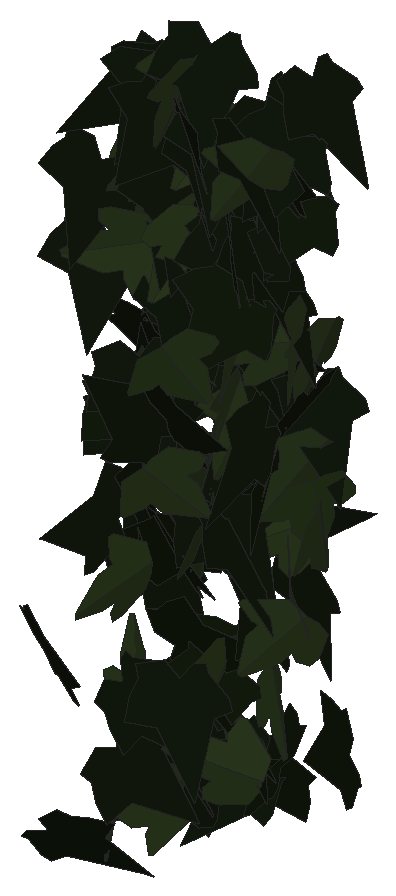
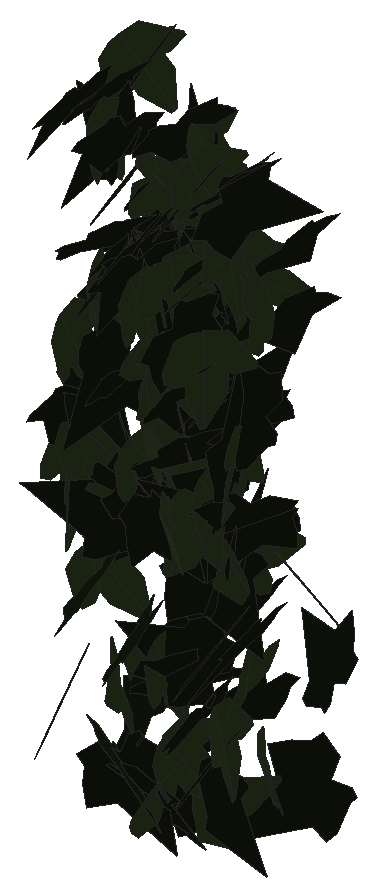
# SketchUp Ruby script. Lengths in inches.
U = 1.inch
M = Sketchup.active_model
def pt(a) = Geom::Point3d.new(a.map { |v| v * U })
def face(e, loops, mat)
  f = e.add_face(loops[0].map { |a| pt(a) })
  loops[1..].each { |l| e.add_face(l.map { |a| pt(a) }).erase! }
  f.material = f.back_material = mat if mat
  f
end
# faces: each face lists its corners as indices into pts; further lists are holes
def faces(e, pts, list, mat = nil) = list.each { |f| face(e, (f[0].is_a?(Array) ? f : [f]).map { |l| l.map { |i| pts[i] } }, mat) }
# xy, xz, yz: faces in a plane at the given z, y or x. An outline is a flat list of corners, or four numbers for a rectangle; further outlines are holes
def ring(l) = l.size == 4 ? [[l[0], l[1]], [l[2], l[1]], [l[2], l[3]], [l[0], l[3]]] : l.each_slice(2).to_a
def flat(e, list, mat, &to3) = list.each { |f| face(e, (f[0].is_a?(Array) ? f : [f]).map { |l| ring(l).map { |u, v| to3.(u, v) } }, mat) }
def xy(e, z, list, mat = nil) = flat(e, list, mat) { |x, y| [x, y, z] }
def xz(e, y, list, mat = nil) = flat(e, list, mat) { |x, z| [x, y, z] }
def yz(e, x, list, mat = nil) = flat(e, list, mat) { |y, z| [x, y, z] }
def lines(e, pts, list) = list.each { |a, b| e.add_line(pt(pts[a]), pt(pts[b])) }
# prism: a flat outline (further loops are holes) pulled along v
def prism(e, loops, v, mat = nil)
  f = face(e, loops, mat); d = Geom::Vector3d.new(v.map { |x| x * U })
  f.pushpull(f.normal.samedirection?(d) ? d.length : -d.length)
end
def box(e, o, s, mat = nil) = prism(e, [[o, [o[0] + s[0], o[1], o[2]], [o[0] + s[0], o[1] + s[1], o[2]], [o[0], o[1] + s[1], o[2]]]], [0, 0, s[2]], mat)
def at(x, y, z, deg = 0) = Geom::Transformation.translation(pt([x, y, z])) * Geom::Transformation.rotation(ORIGIN, Z_AXIS, deg.degrees)
def axes(o, x, y, z) = Geom::Transformation.new([*x, 0, *y, 0, *z, 0, *pt(o).to_a, 1])
def part(name) = M.definitions.add(name)
# library, detail: a bought-in or finely detailed component or shape, given as its bounding box
def library(name, o, s) = part(name).tap { |d| box(d.entities, o, s) }
def detail(e, o, s) = box(e.add_group.entities, o, s)
def put(e, d, t, mat = nil) = e.add_instance(d, t).tap { |i| i.material = mat if mat }
def group(e, t, mat = nil) = e.add_group.tap { |g| g.transformation = t; g.material = mat if mat }.entities
root = M.entities
M.materials.add("efeu1").color = [18, 25, 13]
M.materials.add("efeu2").color = [43, 57, 29]
c1 = part("ivyleaf_10")
p = [[0,0.5,-0.03],[-0.0625,2.02,-0.43],[-0.19,2.01,-0.46],[-0.54,1.05,-0.29],[-0.52,0.625,-0.18],[-0.83,0.76,-0.28],
  [-1.16,0.64,-0.33],[-1.15,0.33,-0.24],[-0.77,-0.39,0.02],[-0.3,-0.51,0.16],[0.04,-0.48,0.23],[-0.02,2.01,-0.4375],
  [-0.06,2.01,-0.43],[0.04,-0.49,0.23],[0.67,-0.49,0.14],[1.38,0.36,-0.2],[1.375,0.51,-0.24],[0.81,0.65,-0.19],
  [0.62,0.59,-0.15],[0.6,1.09,-0.28],[0.5,1.23,-0.31]]
faces(c1.entities,p,[[0,1,2,3,4,5,6,7,8,9,10],[11,12,0,13,14,15,16,17,18,19,20]],"efeu2")
c2 = part("ivyleaf_9")
p = [[1.54,2.16,1.25],[1.36,2.04,1.19],[-0.21,0.99,0.68],[-0.71,1.11,0.82],[-0.85,0.86,0.67],[-0.8,0.17,0.21],
  [-0.9,-0.01,0.1],[-0.67,-0.16,-0.02],[-0.08,-0.08,-0.05],[-0.03,-0.6,-0.4],[0.65,-0.88,-0.66],[0.83,-0.6,-0.49],
  [1.29,-0.42,-0.43],[1.8125,-0.07,-0.26],[1.21,0.44,0.15]]
faces(c2.entities,p,[[0,1,2,3,4,5,6,7,8,9,10,11,12,13,14]],"efeu1")
put(root,c1,axes([24.72,219.9375,231.1],[-0.26803,-0.33753,-0.25345],[0.154,0.20133,-0.43099],[0.39299,-0.3091,-0.00397]))
put(root,c1,axes([24.39,220.07,229.25],[-0.27506,-0.26901,-0.31933],[0.22345,0.22819,-0.38471],[0.35272,-0.35435,-0.00531]))
put(root,c2,axes([22.32,220.66,223.26],[0.44279,0.16175,0.16665],[0.15554,0.0599,-0.4714],[-0.17246,0.46931,0.00273]))
put(root,c2,axes([23.37,220.77,225.64],[0.28987,-0.27115,-0.30406],[-0.10436,0.3113,-0.3771],[0.39381,0.28208,0.12387]))
put(root,c2,axes([21.6875,221.32,225.29],[0.0776,-0.20031,0.4515],[0.2395,-0.38446,-0.21173],[0.43199,0.24913,0.03628]))
put(root,c1,axes([25.07,221.27,233.375],[-0.22833,-0.34455,0.28134],[-0.15546,-0.23449,-0.41334],[0.41677,-0.27623,-0.00005]))
put(root,c1,axes([22.93,221.47,226.76],[0.00446,-0.07801,0.49386],[0.06045,-0.49017,-0.07797],[0.49631,0.0604,0.00506]))
put(root,c2,axes([23.83,221.25,225.61],[-0.01674,-0.48455,-0.12218],[0.021,0.12146,-0.48457],[0.49928,-0.02135,0.01628]))
put(root,c2,axes([23.58,221.36,229.18],[0.12355,-0.17685,0.45106],[0.32099,-0.3188,-0.21291],[0.3629,0.34219,0.03476]))
put(root,c2,axes([23.1,221,224.52],[0.17446,-0.24264,-0.40086],[-0.08105,0.40567,-0.28082],[0.46151,0.16296,0.10222]))
put(root,c2,axes([24.5,221.64,231.04],[-0.28072,-0.37076,0.18367],[-0.04258,-0.19489,-0.45848],[0.41156,-0.27305,0.07785]))
put(root,c1,axes([22.64,221.52,223.77],[0.33246,-0.28404,0.24247],[0.18323,-0.15881,-0.43727],[0.32542,0.37961,-0.0015]))
put(root,c2,axes([24.65,221.48,233.41],[0.22682,-0.44514,0.02016],[0.00787,-0.01862,-0.49959],[0.44552,0.22695,-0.00144]))
put(root,c1,axes([24.58,221.55,224.49],[0.1228,0.09449,0.47539],[-0.36852,-0.30033,0.15489],[0.31482,-0.38842,-0.00412]))
put(root,c2,axes([23.17,221.65,228.72],[0.11074,0.08078,0.48084],[-0.42601,-0.22383,0.13571],[0.23718,-0.43974,0.01926]))
put(root,c2,axes([24.7,221.77,229.23],[-0.45584,0.09514,-0.18209],[0.17798,-0.0385,-0.46566],[-0.10263,-0.48935,0.00123]))
put(root,c1,axes([24.26,221.95,230.53],[0.18839,-0.31913,0.33566],[0.18211,-0.28214,-0.37045],[0.42585,0.26183,0.00993]))
put(root,c1,axes([22.75,221.83,231.16],[0.14923,0.03908,-0.47561],[-0.46455,-0.10214,-0.15416],[-0.1092,0.48789,0.00582]))
put(root,c2,axes([21.92,222.06,231.88],[-0.08745,-0.4731,0.13612],[-0.01255,-0.13606,-0.48097],[0.49213,-0.08754,0.01192]))
put(root,c2,axes([22.05,222.02,230.9],[-0.14558,-0.47731,-0.03131],[0.00828,0.03021,-0.49902],[0.47827,-0.14581,-0.0009]))
put(root,c1,axes([22.84,221.58,224.92],[-0.0429,0.45111,-0.21133],[-0.03949,0.20837,0.4528],[0.49659,0.05554,0.01775]))
put(root,c2,axes([22.43,221.73,227.22],[-0.38421,0.27424,0.16484],[-0.14172,0.08508,-0.47188],[-0.28687,-0.40933,0.01235]))
put(root,c2,axes([24.88,222.22,233.1875],[-0.13675,-0.44013,0.19386],[0.00836,-0.20369,-0.45655],[0.48086,-0.12162,0.06307]))
put(root,c1,axes([22.99,222.2,223.26],[-0.04595,-0.06842,-0.49316],[-0.28888,-0.39971,0.08237],[-0.40551,0.29249,-0.0028]))
put(root,c1,axes([24.61,222.19,230.27],[-0.02582,0.09787,0.48965],[-0.13025,-0.47465,0.088],[0.48205,-0.12301,0.05]))
put(root,c2,axes([24.11,222.12,231.56],[-0.16791,-0.46607,-0.06773],[0.01479,0.06665,-0.49532],[0.47073,-0.16834,-0.00859]))
put(root,c2,axes([23.14,222.25,232.48],[-0.06882,-0.0272,0.49449],[0.16619,-0.47156,-0.00281],[0.46652,0.16397,0.07395]))
put(root,c2,axes([22.5625,222.0625,229.33],[-0.03894,-0.43164,-0.24934],[0.05752,0.24454,-0.43231],[0.49515,-0.06235,0.03061]))
put(root,c2,axes([23.02,222.33,230.36],[0.01714,-0.48179,0.13261],[0.00018,-0.13268,-0.48207],[0.49971,0.01657,-0.00438]))
put(root,c1,axes([23.28,222.18,231.39],[0.29507,0.31806,-0.24854],[-0.16656,-0.1845,-0.43384],[-0.36769,0.33882,-0.00293]))
put(root,c2,axes([22.69,222.45,232.6],[-0.19307,-0.35175,0.29833],[0.00912,-0.32626,-0.37878],[0.46113,-0.14082,0.1324]))
put(root,c2,axes([23.89,222.13,227.47],[0.2481,-0.42833,-0.0706],[-0.02823,0.06522,-0.49492],[0.43319,0.24956,0.00817]))
put(root,c1,axes([24.84,222.23,226.34],[-0.27875,-0.23426,0.34267],[-0.24994,-0.23482,-0.36385],[0.3314,-0.37414,0.01381]))
put(root,c2,axes([24.18,221.83,231.57],[0.15401,0.01023,-0.47558],[-0.45467,0.15013,-0.14401],[0.13985,0.47682,0.05554]))
put(root,c2,axes([22.8,222.32,226.74],[0.16628,-0.25121,0.39906],[0.24177,-0.31787,-0.30084],[0.40484,0.29301,0.01576]))
put(root,c1,axes([24.78,222.39,230.44],[0.116,-0.22516,0.4311],[0.30559,-0.31105,-0.24468],[0.37837,0.32024,0.06545]))
put(root,c2,axes([23.86,222.38,224.46],[0.12444,-0.35426,0.33018],[0.18096,-0.28219,-0.37097],[0.44919,0.21182,0.05799]))
put(root,c2,axes([24.26,222.375,231.38],[0.05809,-0.49218,0.06619],[-0.00237,-0.06692,-0.4955],[0.49661,0.05725,-0.0101]))
put(root,c2,axes([23.12,222.31,231.39],[-0.20092,-0.11777,-0.44245],[0.45268,0.02137,-0.21125],[0.06867,-0.48546,0.09804]))
put(root,c2,axes([24.41,222.375,232.625],[0.11205,-0.16666,0.4579],[0.25785,-0.3784,-0.20082],[0.41347,0.28114,0.00115]))
put(root,c1,axes([23.54,222.08,227.36],[0.1291,-0.45036,-0.17467],[-0.03616,0.17129,-0.46835],[0.48169,0.13356,0.01165]))
put(root,c1,axes([24.13,222.2,231.16],[0.06826,-0.49468,-0.02516],[-0.00314,0.02497,-0.49937],[0.49531,0.06833,0.0003]))
put(root,c2,axes([23.72,222.15,227.61],[-0.12382,-0.22994,-0.42637],[0.23632,0.35549,-0.26034],[0.42288,-0.26599,0.02064]))
put(root,c1,axes([22.97,222.4,233.35],[0.09433,-0.45674,0.18025],[0.03238,-0.17736,-0.46636],[0.48995,0.09966,-0.00388]))
put(root,c2,axes([22.35,222.54,227.24],[-0.02535,0.01442,0.49915],[-0.09722,-0.49037,0.00923],[0.4898,-0.09658,0.02767]))
put(root,c2,axes([22.96,222.29,226.97],[0.06602,0.29946,-0.39492],[-0.11969,-0.37699,-0.30587],[-0.48095,0.13492,0.02191]))
put(root,c2,axes([23.94,222.58,231.35],[-0.24507,-0.41873,0.12087],[-0.0566,-0.10692,-0.48514],[0.43213,-0.25147,0.00501]))
put(root,c2,axes([23.66,222.57,225.15],[-0.34108,-0.11829,0.34594],[-0.28114,-0.21758,-0.35159],[0.23372,-0.43436,0.08191]))
put(root,c2,axes([22.72,222.55,231.72],[-0.04579,-0.49132,0.08066],[0.00115,-0.08111,-0.49338],[0.4979,-0.04499,0.00856]))
put(root,c2,axes([23.08,222.31,223.68],[0.10602,0.07739,-0.48246],[-0.36721,-0.31308,-0.13092],[-0.32236,0.38209,-0.00955]))
put(root,c1,axes([23.58,222.45,225.43],[0.04054,-0.47512,0.15041],[0.03449,-0.14787,-0.47639],[0.49716,0.049,0.02079]))
put(root,c1,axes([24.5625,222.54,232.93],[0.0952,-0.41933,0.25515],[0.1142,-0.23385,-0.42693],[0.47738,0.13957,0.05125]))
put(root,c2,axes([23.2,222.59,232.4],[0.06597,-0.48203,0.11532],[0.03122,-0.11206,-0.48628],[0.49464,0.07136,0.01532]))
put(root,c2,axes([22.97,222.33,225.375],[0.17159,-0.05982,0.46581],[0.42817,-0.18382,-0.18134],[0.19295,0.46112,-0.01186]))
put(root,c2,axes([23.8125,222.39,230.22],[0.26714,-0.41163,-0.09589],[-0.04128,0.08749,-0.49055],[0.42063,0.27001,0.01276]))
put(root,c2,axes([24.37,222.53,230.92],[0.22737,-0.43854,0.07739],[0.04076,-0.06603,-0.49394],[0.44344,0.23092,0.00572]))
put(root,c1,axes([23.63,222.42,232.62],[0.48561,-0.11706,-0.02203],[-0.02105,0.00664,-0.49951],[0.11723,0.48606,0.00152]))
put(root,c1,axes([23.375,222.4,228.29],[0.11573,-0.48503,-0.03674],[-0.01034,0.03531,-0.49864],[0.48631,0.11618,-0.00185]))
put(root,c2,axes([23.41,222.64,232.71],[-0.05821,-0.49347,0.05571],[0.00849,-0.05708,-0.49666],[0.49653,-0.05687,0.01502]))
put(root,c2,axes([24.15,222.54,228.64],[-0.29655,0.04828,-0.39966],[0.39505,-0.06053,-0.30045],[-0.07739,-0.49397,-0.00225]))
put(root,c1,axes([24.9,222.15,226.9],[-0.24302,0.15554,0.40835],[-0.33914,0.2275,-0.28849],[-0.27554,-0.41719,-0.00507]))
put(root,c1,axes([23.23,222.64,224.27],[-0.03149,-0.41545,0.27642],[0.00915,-0.2774,-0.41589],[0.49892,-0.02113,0.02507]))
put(root,c2,axes([22.79,222.74,231.35],[-0.05357,-0.45479,0.20075],[0.05221,-0.20594,-0.45262],[0.49437,-0.02753,0.06955]))
put(root,c1,axes([24.75,222.7,228.53],[-0.0978,-0.35267,0.34068],[-0.07119,-0.33349,-0.36567],[0.48515,-0.12003,0.01502]))
put(root,c1,axes([22.46,222.49,231.96],[-0.08992,-0.49179,0.00755],[-0.00122,-0.00746,-0.49994],[0.49185,-0.08993,0.00014]))
put(root,c1,axes([22.57,222.5,224.8],[0.11796,-0.48463,-0.03495],[-0.00853,0.03389,-0.49878],[0.48581,0.11827,-0.00027]))
put(root,c2,axes([22.95,222.48,224.875],[0.216,-0.41315,-0.18069],[-0.0791,0.16253,-0.46618],[0.44395,0.22997,0.00485]))
put(root,c2,axes([22.34,222.85,232.91],[-0.19327,-0.41326,0.20461],[-0.01051,-0.21785,-0.44992],[0.46102,-0.17821,0.07552]))
put(root,c2,axes([21.95,222.45,229.57],[0.41414,-0.1432,0.2408],[0.22714,-0.07996,-0.43819],[0.16401,0.47234,-0.00118]))
put(root,c1,axes([24.49,222.67,227.42],[-0.23263,-0.00891,0.4425],[-0.34415,-0.31068,-0.18719],[0.27828,-0.39166,0.13842]))
put(root,c2,axes([24.76,222.55,229.36],[-0.22532,0.35938,-0.26472],[0.13684,-0.22665,-0.42415],[-0.42486,-0.26359,0.00379]))
put(root,c2,axes([22.625,222.6,224.3125],[0.22538,-0.44088,-0.0695],[-0.02403,0.06575,-0.49507],[0.44567,0.22651,0.00845]))
put(root,c2,axes([23.11,222.74,233.61],[-0.09058,-0.48867,-0.0547],[0.01088,0.05362,-0.497],[0.49161,-0.09123,0.00092]))
put(root,c1,axes([21.73,222.73,231.39],[-0.01813,0.01684,-0.49939],[0.38062,-0.32329,-0.02472],[-0.32372,-0.38105,-0.00109]))
put(root,c1,axes([24.93,222.51,228.13],[-0.23223,-0.439,-0.05785],[0.01922,0.05527,-0.49656],[0.44238,-0.23286,-0.0088]))
put(root,c2,axes([22.16,222.91,232.85],[-0.0452,-0.1021,-0.48737],[0.05305,-0.48758,0.09722],[-0.49512,-0.04292,0.05491]))
put(root,c2,axes([24.02,222.94,232.31],[-0.07647,-0.3413,0.35731],[0.01507,-0.363,-0.34351],[0.49389,-0.04177,0.0658]))
put(root,c1,axes([23.24,222.58,229.64],[0.23784,-0.43189,-0.08309],[-0.03285,0.07676,-0.49298],[0.43858,0.23996,0.00813]))
put(root,c1,axes([23.33,222.72,232.67],[0.33259,0.25328,-0.27429],[-0.216,-0.16909,-0.41804],[-0.30452,0.39656,-0.00306]))
put(root,c1,axes([23.43,222.82,228.96],[0.1896,-0.40997,0.21443],[0.08069,-0.19889,-0.45159],[0.45557,0.20584,-0.00926]))
put(root,c1,axes([22.5,222.83,228.41],[0.04054,-0.44211,0.22999],[0.03642,-0.2275,-0.44375],[0.49702,0.05273,0.01376]))
put(root,c1,axes([24.96,222.52,227.74],[0.12615,-0.44203,-0.19672],[0.0258,0.20915,-0.45342],[0.48314,0.10425,0.07558]))
put(root,c1,axes([23.99,222.82,225.02],[0.25637,-0.15938,0.39859],[0.37189,-0.14943,-0.29895],[0.21442,0.44974,0.04192]))
put(root,c2,axes([23.62,222.88,227.72],[-0.04613,0.02391,0.49729],[-0.47375,-0.15566,-0.03646],[0.15307,-0.47455,0.03701]))
put(root,c2,axes([23.68,222.85,231.75],[0.10902,-0.48777,0.01412],[-0.00038,-0.01456,-0.49979],[0.48797,0.10896,-0.00354]))
put(root,c2,axes([22.12,222.81,228.79],[0.03635,0.31798,0.38414],[-0.15938,-0.35755,0.31106],[0.47252,-0.14506,0.07537]))
put(root,c2,axes([21.95,222.56,226.5],[0.28285,-0.29675,-0.28624],[-0.10011,0.2873,-0.39678],[0.39996,0.28177,0.10311]))
put(root,c2,axes([24.03,222.73,223.93],[0.15755,0.16235,-0.44589],[-0.29526,-0.33427,-0.22603],[-0.37149,0.33453,-0.00945]))
put(root,c2,axes([22.43,222.75,226.17],[0.25067,-0.42131,-0.09831],[-0.03444,0.09382,-0.48991],[0.43125,0.25238,0.01801]))
put(root,c2,axes([24.1,222.55,227.34],[0.15973,0.01208,0.47365],[0.47363,-0.01746,-0.15928],[0.01269,0.49955,-0.01702]))
put(root,c2,axes([21.99,222.68,228.28],[-0.15499,-0.29184,-0.37524],[0.15834,0.34046,-0.33018],[0.44823,-0.22118,-0.01312]))
put(root,c2,axes([23.8,222.85,223.76],[-0.49962,-0.01108,-0.01617],[0.01619,-0.0008,-0.49974],[0.01105,-0.49988,0.00116]))
put(root,c1,axes([23.55,222.96,228.71],[-0.1326,-0.39992,0.26922],[0.0356,-0.28658,-0.40817],[0.48078,-0.08908,0.10448]))
put(root,c2,axes([23.3125,222.82,230.45],[-0.11718,0.18969,0.44753],[0.18144,-0.41001,0.22129],[0.45094,0.21426,0.02726]))
put(root,c1,axes([24.75,222.92,230.08],[0.05409,-0.45579,0.19832],[0.0437,-0.19436,-0.4586],[0.49514,0.06694,0.01881]))
put(root,c1,axes([23.14,222.8,231.34],[-0.28823,-0.39631,0.09928],[-0.04079,-0.09298,-0.48958],[0.40652,-0.29033,0.02127]))
put(root,c2,axes([21.9,222.78,228.41],[-0.09268,-0.38052,-0.31082],[0.15333,0.27811,-0.38619],[0.4668,-0.16691,0.06514]))
put(root,c1,axes([22.05,222.87,227.34],[0.24622,-0.1711,-0.40013],[0.34167,-0.20871,0.2995],[-0.26951,-0.42091,0.01415]))
put(root,c2,axes([23.69,223.16,225.71],[-0.08565,-0.27815,0.40657],[0.03623,-0.41511,-0.27636],[0.49128,-0.01788,0.09126]))
put(root,c2,axes([23.76,222.76,231.36],[0.07771,-0.42138,-0.25769],[-0.03591,0.25535,-0.42838],[0.49262,0.08508,0.00942]))
put(root,c2,axes([24.94,223.14,224.17],[-0.10209,-0.09661,0.47984],[-0.04885,-0.4857,-0.10819],[0.48702,-0.06897,0.08973]))
put(root,c1,axes([22.18,222.57,229.08],[0.04677,-0.37873,-0.32308],[0.00801,0.32503,-0.37986],[0.49774,0.03035,0.03647]))
put(root,c2,axes([24.08,222.67,233.18],[0.11774,-0.33384,-0.35311],[-0.0436,0.35461,-0.34979],[0.48398,0.11316,0.05439]))
put(root,c2,axes([23.72,223.01,229.91],[-0.02374,-0.49944,0.00044],[-0.00044,-0.00042,-0.5],[0.49944,-0.02374,-0.00042]))
put(root,c1,axes([22.58,222.99,233.1875],[-0.12704,-0.42809,0.22494],[0.02693,-0.23848,-0.43864],[0.48284,-0.09933,0.08365]))
put(root,c2,axes([24.24,223.16,231.71],[-0.2559,-0.40254,0.14992],[0.01228,-0.18129,-0.46581],[0.42938,-0.23472,0.10267]))
put(root,c1,axes([23.5625,222.98,231.01],[0.01024,-0.47245,0.16337],[0.04102,-0.16205,-0.47123],[0.49821,0.02306,0.03544]))
put(root,c2,axes([24.08,222.73,227.81],[-0.44357,-0.10025,-0.20784],[-0.20298,-0.04467,0.45476],[-0.10975,0.48781,-0.00107]))
put(root,c1,axes([23.09,222.66,230.19],[-0.28827,-0.30418,-0.27271],[0.196,0.18988,-0.41897],[0.35845,-0.34845,0.00977]))
put(root,c1,axes([23.22,222.77,230.13],[-0.38771,-0.28773,-0.12996],[0.10216,0.08041,-0.4828],[0.29874,-0.40093,-0.00356]))
put(root,c2,axes([23.32,222.99,228.08],[-0.13801,0.29639,-0.3783],[0.16599,-0.33997,-0.32691],[-0.451,-0.21582,-0.00456]))
put(root,c1,axes([22.92,223.01,230.37],[-0.19142,-0.42621,0.17805],[-0.0176,-0.18586,-0.46384],[0.46157,-0.18384,0.05615]))
put(root,c1,axes([22.7,222.8125,227.95],[-0.45793,0.0901,-0.17941],[0.17618,-0.03385,-0.4667],[-0.09625,-0.49065,-0.00075]))
put(root,c2,axes([22.71,223.03,229.99],[-0.01102,-0.4935,-0.0796],[-0.00811,0.07978,-0.49353],[0.49981,-0.00959,-0.00976]))
put(root,c2,axes([24.23,222.67,223.96],[-0.26594,0.35127,0.2364],[-0.14939,0.18336,-0.44052],[-0.39618,-0.30494,0.00743]))
put(root,c1,axes([23.34,223.14,223.51],[-0.19181,0.26097,0.38092],[0.07764,-0.38838,0.30518],[0.45517,0.17622,0.10847]))
put(root,c2,axes([24.6,222.93,229.23],[-0.00827,-0.45288,-0.21173],[-0.00479,0.21182,-0.45289],[0.49991,-0.00546,-0.00784]))
put(root,c2,axes([22.97,223.24,228.98],[-0.28253,-0.35222,0.21474],[-0.06105,-0.22171,-0.44398],[0.40798,-0.2771,0.08227]))
put(root,c2,axes([22.625,223.16,232.84],[0.07278,-0.47247,0.14655],[0.02414,-0.14456,-0.47804],[0.49409,0.07665,0.00177]))
put(root,c2,axes([24.65,222.875,233.62],[0.19197,-0.41216,-0.20803],[-0.03979,0.20969,-0.45216],[0.45996,0.19015,0.04771]))
put(root,c1,axes([22.98,223.1,227.91],[0.28462,-0.30224,0.27864],[0.19287,-0.20111,-0.41516],[0.36303,0.34381,0.00211]))
put(root,c2,axes([22.77,223.22,230.89],[-0.00951,0.05314,-0.49708],[0.18672,-0.46081,-0.05283],[-0.46373,-0.18664,-0.01108]))
put(root,c2,axes([23.99,222.71,229.82],[0.48184,0.10836,-0.07801],[-0.07736,-0.01156,-0.49384],[-0.10883,0.48798,0.00562]))
put(root,c1,axes([22.54,222.92,230.53],[-0.28439,-0.41109,-0.0114],[0.01053,0.00658,-0.49985],[0.41111,-0.28454,0.00492]))
put(root,c2,axes([24.26,223.125,226.5],[0.19162,-0.44914,0.10749],[0.04126,-0.09927,-0.48831],[0.45998,0.19601,-0.00098]))
